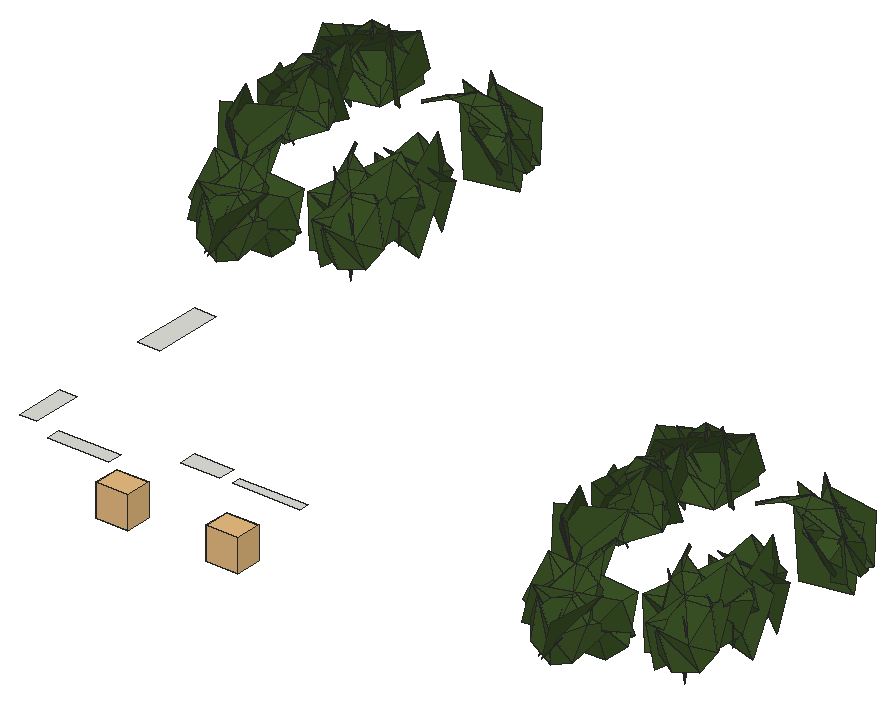
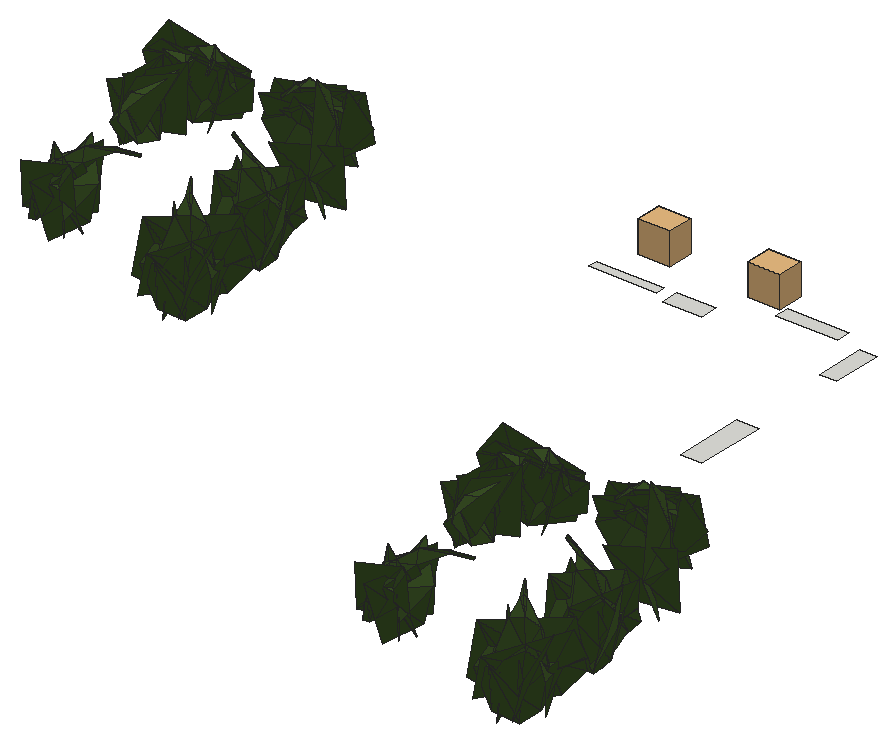
# SketchUp Ruby script. Lengths in inches.
U = 1.inch
M = Sketchup.active_model
def pt(a) = Geom::Point3d.new(a.map { |v| v * U })
def face(e, loops, mat)
  f = e.add_face(loops[0].map { |a| pt(a) })
  loops[1..].each { |l| e.add_face(l.map { |a| pt(a) }).erase! }
  f.material = f.back_material = mat if mat
  f
end
# faces: each face lists its corners as indices into pts; further lists are holes
def faces(e, pts, list, mat = nil) = list.each { |f| face(e, (f[0].is_a?(Array) ? f : [f]).map { |l| l.map { |i| pts[i] } }, mat) }
# xy, xz, yz: faces in a plane at the given z, y or x. An outline is a flat list of corners, or four numbers for a rectangle; further outlines are holes
def ring(l) = l.size == 4 ? [[l[0], l[1]], [l[2], l[1]], [l[2], l[3]], [l[0], l[3]]] : l.each_slice(2).to_a
def flat(e, list, mat, &to3) = list.each { |f| face(e, (f[0].is_a?(Array) ? f : [f]).map { |l| ring(l).map { |u, v| to3.(u, v) } }, mat) }
def xy(e, z, list, mat = nil) = flat(e, list, mat) { |x, y| [x, y, z] }
def xz(e, y, list, mat = nil) = flat(e, list, mat) { |x, z| [x, y, z] }
def yz(e, x, list, mat = nil) = flat(e, list, mat) { |y, z| [x, y, z] }
def lines(e, pts, list) = list.each { |a, b| e.add_line(pt(pts[a]), pt(pts[b])) }
# prism: a flat outline (further loops are holes) pulled along v
def prism(e, loops, v, mat = nil)
  f = face(e, loops, mat); d = Geom::Vector3d.new(v.map { |x| x * U })
  f.pushpull(f.normal.samedirection?(d) ? d.length : -d.length)
end
def box(e, o, s, mat = nil) = prism(e, [[o, [o[0] + s[0], o[1], o[2]], [o[0] + s[0], o[1] + s[1], o[2]], [o[0], o[1] + s[1], o[2]]]], [0, 0, s[2]], mat)
def at(x, y, z, deg = 0) = Geom::Transformation.translation(pt([x, y, z])) * Geom::Transformation.rotation(ORIGIN, Z_AXIS, deg.degrees)
def axes(o, x, y, z) = Geom::Transformation.new([*x, 0, *y, 0, *z, 0, *pt(o).to_a, 1])
def part(name) = M.definitions.add(name)
# library, detail: a bought-in or finely detailed component or shape, given as its bounding box
def library(name, o, s) = part(name).tap { |d| box(d.entities, o, s) }
def detail(e, o, s) = box(e.add_group.entities, o, s)
def put(e, d, t, mat = nil) = e.add_instance(d, t).tap { |i| i.material = mat if mat }
def group(e, t, mat = nil) = e.add_group.tap { |g| g.transformation = t; g.material = mat if mat }.entities
root = M.entities
M.materials.add("AM113_062_Tilia").color = [58, 81, 37]
c1 = library("Plante \#58",[-0.43,-1.58,0],[20.84,18.06,17.59])
xy(root,249.78,[[496.21,121.6875,613.65,148.5625],[418.81,151.95,449.99,247.52],[699,187.1875,773.61,220.1875],[798.31,187.1875,927.68,205.0625],[418.81,435.18,460.62,569.75]])
p = [[1401.53,610.83,371.375],[1421.48,599.4,247.5625],[1379.93,662.74,198.97],[1327.42,667.66,291.15],[240.9,1259.61,371.375],[260.86,1248.18,247.5625],
  [219.3,1311.51,198.97],[166.79,1316.43,291.15],[1297.48,648.87,290.96],[1328.96,610.16,204.4],[1335.8,554.83,274.0625],[136.85,1297.64,290.96],
  [168.34,1258.93,204.4],[175.17,1203.6,274.0625],[1491.89,98.47,290.2],[1465.99,189.64,367.67],[1437.45,123.25,205.52],[1438.65,201.7,246.33],
  [331.26,747.24,290.2],[305.36,838.41,367.67],[276.82,772.03,205.52],[278.02,850.48,246.33],[1337.9375,661.05,211.125],[1317.23,635.33,228.34],
  [1334.6,667.78,260.74],[1384.17,678.53,300.4],[1374.32,682.52,229.72],[177.3125,1309.82,211.125],[156.6,1284.11,228.34],[173.97,1316.56,260.74],
  [223.54,1327.31,300.4],[213.6875,1331.29,229.72],[1475.88,104.4,211.61],[1481.79,100.05,261.27],[1439.04,118.16,308.89],[1508.34,117.24,220.77],
  [1436.59,105.34,238.88],[315.25,753.18,211.61],[321.17,748.83,261.27],[278.42,766.9375,308.89],[347.71,766.02,220.77],[275.96,754.11,238.88],
  [1618.27,508.73,357.65],[1627.9,508.43,230.94],[1697.68,554.0625,212.5],[1686.84,591.33,315.55],[457.64,1157.51,357.65],[467.27,1157.2,230.94],
  [537.06,1202.84,212.5],[526.22,1240.1,315.55],[1458.17,154.61,217.56],[1531.51,166.52,212.64],[1523.46,146.3125,289.33],[1575.21,164.51,251.43],
  [297.54,803.39,217.56],[370.88,815.29,212.64],[362.83,795.09,289.33],[414.59,813.29,251.43],[1293.25,457.23,296.9],[1344.65,453.13,214.11],
  [1374.94,400.81,274.41],[132.62,1106.01,296.9],[184.03,1101.9,214.11],[214.32,1049.58,274.41],[1668.4,621.42,317.93],[1645.21,605.22,216.42],
  [1579.5625,590.09,266.15],[507.77,1270.2,317.93],[484.58,1253.99,216.42],[418.9375,1238.87,266.15],[1692.14,158.89,327.71],[1606.23,223.25,369.83],
  [1675.86,176.32,217.35],[1630.35,243.26,249.11],[531.51,807.67,327.71],[445.6,872.03,369.83],[515.23,825.1,217.35],[469.72,892.03,249.11],
  [1421.47,168.41,360.97],[1399.97,130.95,286.27],[1468.42,133.77,299.82],[260.84,817.18,360.97],[239.35,779.72,286.27],[307.79,782.55,299.82],
  [1378.82,627.1,218.48],[1321.4,580.7,230.41],[1324.24,611.04,301.99],[1366.06,649.77,299.33],[1428.59,649.92,353.15],[1422.36,683.8,271.24],
  [218.19,1275.875,218.48],[160.77,1229.47,230.41],[163.61,1259.82,301.99],[205.43,1298.55,299.33],[267.96,1298.69,353.15],[261.73,1332.58,271.24],
  [1527.38,129.19,287.65],[1554.9,169.94,286.05],[366.75,777.96,287.65],[394.28,818.71,286.05],[1336.2,596.66,325.1],[1318,605.13,346.58],
  [1339.6,676.65,221.31],[1359.41,648.01,226.7],[1312.01,684.67,303.7],[175.57,1245.43,325.1],[157.375,1253.9,346.58],[178.98,1325.43,221.31],
  [198.79,1296.79,226.7],[151.39,1333.45,303.7],[1659.6,483.47,343.94],[1706.36,500.69,276.47],[1659.62,553.57,221.6875],[1668.18,552.92,308.53],
  [1629.73,595,311.23],[1612.0625,609.82,235.1875],[498.98,1132.24,343.94],[545.73,1149.47,276.47],[498.99,1202.35,221.6875],[507.55,1201.69,308.53],
  [469.11,1243.77,311.23],[451.44,1258.6,235.1875],[1701.93,523.76,332],[1713.14,518.09,250.46],[1638.7,545.04,221.76],[1678.83,572.46,283.6875],
  [1589.21,594.72,243.73],[1632.9375,605.61,301.24],[541.31,1172.54,332],[552.51,1166.86,250.46],[478.07,1193.81,221.76],[518.2,1221.23,283.6875],
  [428.58,1243.5,243.73],[472.31,1254.38,301.24],[1431.0625,114.96,330.64],[1406.36,121.03,254.26],[1461.84,176.5625,222.62],[1474.8,119.35,267.77],
  [1528.86,140.13,275.47],[1532.21,191.88,228.45],[270.43,763.74,330.64],[245.73,769.81,254.26],[301.21,825.34,222.62],[314.17,768.125,267.77],
  [368.23,788.91,275.47],[371.59,840.66,228.45],[1537.35,151.08,331.19],[1498.47,76.875,303.85],[1468.18,92.44,224.9],[1465.74,127.39,227.19],
  [1523.1,166.15,310.81],[376.73,799.86,331.19],[337.84,725.65,303.85],[307.55,741.22,224.9],[305.11,776.16,227.19],[362.47,814.93,310.81],
  [1387.08,607.01,226.52],[1334.77,560.38,248.76],[1315.4,612.11,288.86],[1350.81,655.32,267.67],[1391.14,687.72,319.77],[1409.37,685.47,240.08],
  [226.45,1255.79,226.52],[174.15,1209.15,248.76],[154.77,1260.89,288.86],[190.18,1304.1,267.67],[230.51,1336.5,319.77],[248.75,1334.25,240.08],
  [1308.45,487.72,306.09],[1394.97,466.23,390.24],[1360.18,522.91,227.3],[1424.8,484.26,273.24],[147.82,1136.49,306.09],[234.34,1115.01,390.24],
  [199.56,1171.68,227.3],[264.18,1133.04,273.24],[1308.82,575.06,307.89],[1312.15,623.6875,299.37],[148.2,1223.83,307.89],[151.52,1272.46,299.37],
  [1577.04,179.99,263.91],[416.42,828.76,263.91],[1417.83,672.38,286.53],[257.21,1321.16,286.53],[1325.35,498.83,230.09],[1320.41,464.74,238.56],
  [1316.16,495.71,278.26],[1349.57,523.74,328.36],[1343.44,532.14,258.76],[164.72,1147.61,230.09],[159.78,1113.52,238.56],[155.53,1144.49,278.26],
  [188.9375,1172.51,328.36],[182.81,1180.92,258.76],[1285.92,565.8,277.58],[125.29,1214.57,277.58],[1352.1,421.25,233.21],[1327.48,384.51,269.14],
  [1334.52,437.67,307.38],[1376.59,490.05,240.53],[191.47,1070.03,233.21],[166.85,1033.29,269.14],[173.89,1086.44,307.38],[215.96,1138.83,240.53],
  [1743.65,305.89,338.78],[1640.54,277.08,382.07],[1728.97,273.24,233.93],[1646,276.04,254.96],[583.03,954.66,338.78],[479.91,925.85,382.07],
  [568.34,922.01,233.93],[485.375,924.82,254.96],[1693.82,593.43,234.48],[1692.08,588.9,284.64],[1696.16,533.89,312.75],[1711.83,554.125,248.77],
  [1665.74,612.11,249.24],[533.1875,1242.2,234.48],[531.45,1237.68,284.64],[535.54,1182.67,312.75],[551.2,1202.9,248.77],[505.11,1260.88,249.24],
  [1589.47,638.01,285.37],[428.84,1286.78,285.37],[1623.09,148.125,316.76],[1633.16,156.84,235.42],[1667.21,231.15,247.11],[462.47,796.9,316.76],
  [472.53,805.62,235.42],[506.58,879.92,247.11],[1339.98,399.32,304.49],[1318.03,442.49,304.26],[179.35,1048.09,304.49],[157.41,1091.26,304.26],
  [1411.35,139.47,298.47],[250.72,788.25,298.47],[1328.75,294.88,354.19],[1425.77,351.23,352.55],[1329.97,285.96,240.22],[1412.67,303.7,242.26],
  [168.125,943.66,354.19],[265.14,1000.01,352.55],[169.34,934.73,240.22],[252.05,952.48,242.26],[1707.36,589.64,248.06],[1678.58,570.53,240.28],
  [1611.88,580.33,326.33],[546.73,1238.42,248.06],[517.95,1219.3,240.28],[451.25,1229.1,326.33],[1349.44,491.01,319.28],[1398.32,514.71,384.12],
  [1380.375,551.29,308.92],[188.82,1139.79,319.28],[237.7,1163.49,384.12],[219.75,1200.07,308.92],[1583.14,189.92,332.99],[1611.48,159.19,256.98],
  [1674.81,210.39,241.09],[1656.96,182.38,317.4375],[1698.36,213.68,347.96],[1728.11,246.31,289.44],[422.51,838.69,332.99],[450.85,807.97,256.98],
  [514.18,859.16,241.09],[496.33,831.16,317.4375],[537.73,862.45,347.96],[567.48,895.08,289.44],[1329.76,423.34,348.22],[1286.05,492.35,317.56],
  [1318.05,511.15,242.59],[1350.58,428.44,329.99],[1349.09,496.53,247.59],[169.14,1072.11,348.22],[125.42,1141.13,317.56],[157.42,1159.93,242.59],
  [189.96,1077.22,329.99],[188.46,1145.31,247.59],[1746.25,340.96,343.3125],[1716.22,345.14,242.78],[1654.94,369.13,295.86],[585.625,989.74,343.3125],
  [555.6,993.92,242.78],[494.32,1017.91,295.86],[1574.67,629.3,293.6875],[414.04,1278.08,293.6875],[1636.83,156.92,304.37],[1611.92,169.03,274.97],
  [1668.39,154.5625,245.06],[1709.77,170.67,250.82],[476.2,805.7,304.37],[451.29,817.8,274.97],[507.76,803.34,245.06],[549.14,819.45,250.82],
  [1659.15,233.05,365.03],[1706.01,222.42,295.4375],[1697.92,294.62,245.38],[1705.99,285.8125,331.56],[1699.33,342.24,338.03],[1692.31,367.44,263.67],
  [498.53,881.82,365.03],[545.38,871.2,295.4375],[537.29,943.39,245.38],[545.36,934.59,331.56],[538.7,991.01,338.03],[531.68,1016.22,263.67],
  [1342.18,359.25,321.77],[1331.32,334.7,246.19],[1387.98,275.52,255.41],[181.55,1008.02,321.77],[170.7,983.47,246.19],[227.35,924.29,255.41],
  [1716.82,241.62,351.96],[1721.21,233.59,269.66],[1675.95,299.85,246.41],[1725.6,296.43,306.79],[1707.94,349.37,328.23],[1665.09,368.14,273.05],
  [556.1875,890.39,351.96],[560.58,882.37,269.66],[515.33,948.625,246.41],[564.97,945.21,306.79],[547.32,998.15,328.23],[504.46,1016.91,273.05],
  [1393.42,476.38,246.98],[1372.7,408.48,250.62],[1327.37,436.01,293.05],[1335.72,492.49,286.42],[1349.47,532.09,349.86],[1370.52,550.61,276.4375],
  [232.79,1125.16,246.98],[212.07,1057.26,250.62],[166.74,1084.78,293.05],[175.09,1141.27,286.42],[188.84,1180.86,349.86],[209.89,1199.39,276.4375],
  [1680.36,175.87,296.02],[1710.47,211.78,340.59],[1712.5625,267.67,302.1],[519.73,824.64,296.02],[549.84,860.56,340.59],[551.9375,916.44,302.1],
  [1616.48,594.5625,353.88],[1701.29,603.85,336.18],[455.85,1243.34,353.88],[540.67,1252.63,336.18],[1692.63,503.25,289.13],[1293.1,553.06,291.86],
  [532,1152.03,289.13],[132.47,1201.83,291.86],[1642.47,606.75,315.3],[1593.54,610.6,311],[481.84,1255.53,315.3],[432.92,1259.38,311],
  [1339.23,375.51,282.48],[178.6,1024.28,282.48],[1695.66,161.29,296.4],[1725.86,191.9,281.32],[535.03,810.0625,296.4],[565.23,840.67,281.32],
  [1563.02,203.66,323.875],[402.4,852.43,323.875],[1414.51,228.18,316.78],[1372.08,258.7,363.04],[1342.47,293.73,316.78],[253.88,876.96,316.78],
  [211.45,907.47,363.04],[181.84,942.51,316.78],[1381.625,537.4,321.02],[221,1186.18,321.02],[1341.59,642.15,326.9],[180.96,1290.93,326.9],
  [1496.63,129.79,322.2],[336.01,778.57,322.2],[1691.24,401.56,316.12],[530.62,1050.33,316.12],[1567.46,161.01,328.74],[406.84,809.79,328.74],
  [1600.42,528.37,350.8125],[439.79,1177.15,350.8125],[1363.05,376.12,343.81],[202.42,1024.9,343.81],[1674.29,402.77,325.01],[513.66,1051.55,325.01],
  [1383.27,591.51,364.84],[222.64,1240.29,364.84],[1390.15,442.03,377.27],[229.52,1090.81,377.27],[1611,213.61,325.14],[450.37,862.39,325.14],
  [1321.75,546.54,350.32],[161.125,1195.3125,350.32],[1331.38,468.58,339.66],[170.76,1117.36,339.66],[1708.53,199.38,350.03],[1714.66,246.375,367.02],
  [547.9,848.16,350.03],[554.03,895.15,367.02],[1324.0625,392.68,345.17],[163.4375,1041.46,345.17],[1656.02,573,339.11],[495.4,1221.78,339.11],
  [1558.66,592.6,340.46],[398.03,1241.375,340.46],[1516.48,189.14,306.09],[355.85,837.92,306.09],[1409.9,623.9,329.08],[249.28,1272.68,329.08],
  [1516.09,170.28,335.125],[355.47,819.05,335.125],[1296.93,581.68,351.58],[136.3,1230.46,351.58],[1638.14,506.44,318.61],[477.52,1155.22,318.61],
  [1746.3,253.16,353.17],[585.67,901.93,353.17],[1592.66,615.36,357.68],[432.03,1264.14,357.68],[1637.36,303.67,377],[476.74,952.44,377],
  [1670.8,184.71,356.48],[510.18,833.49,356.48],[1447.08,179.92,329.75],[286.45,828.7,329.75],[1353.05,579.51,321.47],[1346.21,599.37,347.96],
  [192.42,1228.29,321.47],[185.58,1248.14,347.96],[1390.375,621.98,357.13],[229.75,1270.76,357.13],[1736.72,266.23,364.25],[576.1,915.01,364.25],
  [1373.73,423.16,327.4],[1356.18,432.44,354.51],[213.11,1071.93,327.4],[195.55,1081.22,354.51],[1619.55,211.1,361.13],[458.93,859.875,361.13],
  [1468.35,173.54,354.39],[307.73,822.32,354.39],[1595.82,565.03,313.82],[435.19,1213.81,313.82],[1631.49,521.39,349.95],[470.86,1170.17,349.95],
  [1610.75,566.94,346.36],[450.12,1215.72,346.36],[1640.7,380.5,371.4],[480.07,1029.27,371.4],[1710.18,235.98,411.79],[1415.91,216.4,384.62],
  [549.56,884.75,411.79],[255.28,865.17,384.62],[1397.65,487.24,353.14],[237.03,1136.01,353.14],[1407.13,259.51,426.27],[246.5,908.28,426.27],
  [1494.76,166.66,357.21],[334.13,815.43,357.21],[1681.88,378.57,387.34],[521.25,1027.34,387.34],[1364.46,615.44,364.78],[203.84,1264.22,364.78],
  [1380.72,471.92,375.875],[220.1,1120.7,375.875],[1692.61,274.66,402.96],[531.98,923.44,402.96],[1490.66,213.67,362.69],[330.03,862.45,362.69],
  [1623.71,545.875,362.15],[463.08,1194.65,362.15],[1362.07,452.49,376.91],[201.44,1101.27,376.91],[1589.59,517,358.89],[1556.77,494.82,348.58],
  [1558.61,494.06,343.77],[1595.07,514.69,353.97],[1585.29,518.92,353.72],[1557.06,496.53,343.78],[428.96,1165.78,358.89],[396.14,1143.6,348.58],
  [397.98,1142.83,343.77],[434.44,1163.47,353.97],[424.66,1167.7,353.72],[396.4375,1145.3,343.78],[1392.01,577.58,374.22],[231.38,1226.36,374.22],
  [1664.98,226.66,379.7],[1669.95,248.51,355.21],[504.35,875.4375,379.7],[509.33,897.29,355.21],[1482.18,207.26,363.76],[321.55,856.04,363.76],
  [1404.1,433.52,386.03],[243.48,1082.3,386.03],[1641.1,213.02,382.77],[480.48,861.8,382.77],[1396.16,587.34,372.8],[235.53,1236.12,372.8],
  [1487.76,210.08,368.01],[327.14,858.86,368.01],[1613.45,245.46,377.6],[452.83,894.24,377.6],[1484.42,250.33,369.4],[1484.84,250.04,364.14],
  [323.79,899.11,369.4],[324.21,898.8125,364.14],[1482,249.89,364.96],[321.37,898.66,364.96],[1393.11,582.71,378.46],[232.48,1231.48,378.46],
  [1417.79,550.86,378.4],[257.17,1199.64,378.4],[1415.36,549.26,378.22],[1416.29,549.83,383.33],[254.74,1198.04,378.22],[255.66,1198.6,383.33],
  [1402.59,443.88,386.99],[241.96,1092.65,386.99],[1596.65,284.64,376.87],[1614.9,249.28,385.05],[1596.51,285.2,382.27],[1402.11,437.72,391.11],
  [436.02,933.42,376.87],[454.27,898.06,385.05],[435.88,933.97,382.27],[241.49,1086.49,391.11],[1617.91,254.34,382.59],[1599.09,285.84,378.24],
  [457.28,903.12,382.59],[438.46,934.61,378.24],[1438.02,421.14,390.46],[1438.2,421.35,395.66],[277.39,1069.91,390.46],[277.57,1070.12,395.66],
  [1439.2,423.65,391.38],[278.58,1072.43,391.38]]
faces(root,p,[[0,1,2],[3,0,2],[4,5,6],[7,4,6],[8,9,10],[11,12,13],[14,15,16],[15,17,16],
  [18,19,20],[19,21,20],[22,23,24],[22,24,25],[25,26,22],[27,28,29],[27,29,30],[30,31,27],
  [32,33,34],[32,35,33],[34,36,32],[37,38,39],[37,40,38],[39,41,37],[42,43,44],[45,42,44],
  [46,47,48],[49,46,48],[50,51,52],[51,53,52],[54,55,56],[55,57,56],[58,59,60],[61,62,63],
  [64,65,66],[67,68,69],[70,71,72],[71,73,72],[74,75,76],[75,77,76],[78,79,50],[50,80,78],
  [52,80,50],[81,82,54],[54,83,81],[56,83,54],[84,85,86],[86,87,84],[84,87,88],[88,89,84],
  [90,91,92],[92,93,90],[90,93,94],[94,95,90],[33,35,96],[35,97,96],[38,40,98],[40,99,98],
  [100,101,102],[102,103,100],[101,104,102],[105,106,107],[107,108,105],[106,109,107],[110,111,112],[112,113,110],
  [114,113,112],[112,115,114],[116,117,118],[118,119,116],[120,119,118],[118,121,120],[122,123,124],[124,125,122],
  [124,126,127],[127,125,124],[128,129,130],[130,131,128],[130,132,133],[133,131,130],[134,135,136],[136,137,134],
  [138,137,136],[136,139,138],[140,141,142],[142,143,140],[144,143,142],[142,145,144],[146,147,148],[148,149,150],
  [150,146,148],[151,152,153],[153,154,155],[155,151,153],[156,157,158],[158,159,156],[156,159,160],[160,161,156],
  [162,163,164],[164,165,162],[162,165,166],[166,167,162],[168,169,170],[169,171,170],[172,173,174],[173,175,174],
  [23,176,177],[24,23,177],[28,178,179],[29,28,179],[139,180,138],[145,181,144],[25,182,26],[30,183,31],
  [184,185,186],[184,186,187],[187,188,184],[189,190,191],[189,191,192],[192,193,189],[85,194,86],[91,195,92],
  [196,197,198],[199,196,198],[200,201,202],[203,200,202],[204,205,206],[205,207,206],[208,209,210],[209,211,210],
  [212,213,214],[214,215,212],[212,216,213],[217,218,219],[219,220,217],[217,221,218],[115,222,114],[121,223,120],
  [224,225,226],[227,228,229],[185,230,231],[186,185,231],[190,232,233],[191,190,233],[34,234,36],[39,235,41],
  [236,237,238],[237,239,238],[240,241,242],[241,243,242],[244,245,246],[247,248,249],[198,250,199],[199,250,251],
  [251,252,199],[202,253,203],[203,253,254],[254,255,203],[256,257,258],[258,259,256],[260,259,258],[258,261,260],
  [262,263,264],[264,265,262],[266,265,264],[264,267,266],[268,269,270],[271,268,270],[270,272,271],[273,274,275],
  [276,273,275],[275,277,276],[278,279,280],[281,282,283],[126,284,127],[132,285,133],[286,287,288],[286,288,289],
  [290,291,292],[290,292,293],[294,295,296],[296,297,294],[298,297,296],[296,299,298],[300,301,302],[302,303,300],
  [304,303,302],[302,305,304],[306,307,308],[309,310,311],[312,313,314],[314,315,312],[316,315,314],[314,317,316],
  [318,319,320],[320,321,318],[322,321,320],[320,323,322],[324,325,326],[326,327,324],[324,327,328],[328,329,324],
  [330,331,332],[332,333,330],[330,333,334],[334,335,330],[226,336,224],[337,336,226],[226,338,337],[229,339,227],
  [340,339,229],[229,341,340],[246,342,244],[342,343,244],[249,344,247],[344,345,247],[214,346,215],[157,347,158],
  [219,348,220],[163,349,164],[213,216,350],[216,351,350],[218,221,352],[221,353,352],[325,354,326],[331,355,332],
  [289,356,286],[289,357,356],[293,358,290],[293,359,358],[52,53,360],[56,57,361],[308,362,363],[363,364,308],
  [308,364,306],[311,365,366],[366,367,311],[311,367,309],[187,368,188],[192,369,193],[370,24,177],[25,24,370],
  [371,29,179],[30,29,371],[34,33,372],[372,33,96],[39,38,373],[373,38,98],[299,374,298],[305,375,304],
  [138,180,376],[144,181,377],[64,66,378],[67,69,379],[160,159,158],[166,165,164],[134,137,138],[140,143,144],
  [198,197,380],[202,201,381],[317,382,316],[323,383,322],[8,10,384],[11,13,385],[58,60,386],[61,63,387],
  [388,287,286],[389,291,290],[138,376,134],[144,377,140],[86,194,390],[92,195,391],[392,186,231],[187,186,392],
  [393,191,233],[192,191,393],[356,357,394],[357,395,394],[358,359,396],[359,397,396],[326,354,398],[332,355,399],
  [122,125,127],[128,131,133],[214,213,400],[400,213,350],[219,218,401],[401,218,352],[114,222,402],[120,223,403],
  [96,97,404],[98,99,405],[328,327,326],[334,333,332],[406,182,25],[407,183,30],[372,96,408],[404,408,96],
  [373,98,409],[405,409,98],[158,347,410],[158,410,160],[164,349,411],[164,411,166],[412,346,214],[413,348,219],
  [78,80,52],[52,360,78],[81,83,56],[56,361,81],[261,414,260],[267,415,266],[326,398,328],[332,399,334],
  [127,284,416],[133,285,417],[278,280,418],[281,283,419],[224,336,337],[227,339,340],[286,356,420],[420,356,394],
  [290,358,421],[421,358,396],[422,234,34],[423,235,39],[88,87,86],[94,93,92],[177,176,424],[424,425,177],
  [370,177,425],[179,178,426],[426,427,179],[371,179,427],[428,25,370],[25,428,406],[429,30,371],[30,429,407],
  [127,416,122],[133,417,128],[86,390,88],[92,391,94],[338,430,337],[341,431,340],[231,230,432],[432,433,231],
  [392,231,433],[233,232,434],[434,435,233],[393,233,435],[286,436,388],[436,286,420],[290,437,389],[437,290,421],
  [312,315,316],[318,321,322],[198,380,251],[251,250,198],[202,381,254],[254,253,202],[110,113,114],[116,119,120],
  [34,438,422],[438,34,372],[39,439,423],[439,39,373],[350,351,440],[352,353,441],[114,402,110],[120,403,116],
  [214,442,412],[442,214,400],[219,443,413],[443,219,401],[440,444,350],[441,445,352],[400,350,444],[401,352,445],
  [298,374,446],[304,375,447],[337,448,224],[362,449,363],[306,364,363],[340,450,227],[365,451,366],[309,367,366],
  [256,259,260],[262,265,266],[452,368,187],[453,369,192],[363,454,306],[366,455,309],[372,456,438],[372,408,456],
  [373,457,439],[373,409,457],[316,382,458],[322,383,459],[370,425,460],[370,460,428],[371,427,461],[371,461,429],
  [316,458,312],[322,459,318],[462,187,392],[187,462,452],[463,192,393],[192,463,453],[294,297,298],[300,303,304],
  [260,464,256],[266,465,262],[456,408,466],[457,409,467],[298,446,294],[304,447,300],[400,468,442],[400,444,468],
  [401,469,443],[401,445,469],[392,433,470],[392,470,462],[393,435,471],[393,471,463],[337,430,448],[340,431,450],
  [472,473,474],[474,475,472],[476,477,473],[478,479,480],[480,481,478],[482,483,479],[468,444,476],[469,445,482],
  [260,414,464],[460,425,484],[266,415,465],[461,427,485],[473,472,476],[479,478,482],[475,442,468],[481,443,469],
  [420,394,486],[487,486,394],[394,395,487],[421,396,488],[489,488,396],[396,397,489],[476,472,468],[482,478,469],
  [468,472,475],[469,478,481],[490,438,456],[491,439,457],[470,433,492],[471,435,493],[420,494,436],[420,486,494],
  [421,495,437],[421,488,495],[496,428,460],[497,429,461],[456,498,490],[466,498,456],[457,499,491],[467,499,457],
  [500,436,494],[501,437,495],[502,498,466],[466,503,502],[504,499,467],[467,505,504],[363,449,454],[366,451,455],
  [506,490,498],[507,491,499],[484,508,460],[460,508,496],[485,509,461],[461,509,497],[498,502,506],[499,504,507],
  [510,496,508],[511,497,509],[484,512,513],[513,508,484],[485,514,515],[515,509,485],[516,462,470],[517,463,471],
  [518,500,519],[519,520,518],[492,521,470],[470,521,516],[522,501,523],[523,524,522],[493,525,471],[471,525,517],
  [494,519,500],[495,523,501],[526,527,520],[528,529,524],[508,513,510],[509,515,511],[494,486,526],[495,488,528],
  [520,519,526],[524,523,528],[526,519,494],[528,523,495],[492,530,531],[531,521,492],[493,532,533],[533,525,493],
  [534,516,521],[535,517,525],[521,531,534],[525,533,535]],"AM113_062_Tilia")
put(root,c1,axes([663.81,32.98,211.83],[2.9928,0,0],[0,2.7666,0],[0,0,3.48]))
put(root,c1,axes([874.84,32.98,211.83],[2.9928,0,0],[0,2.7666,0],[0,0,3.48]))
